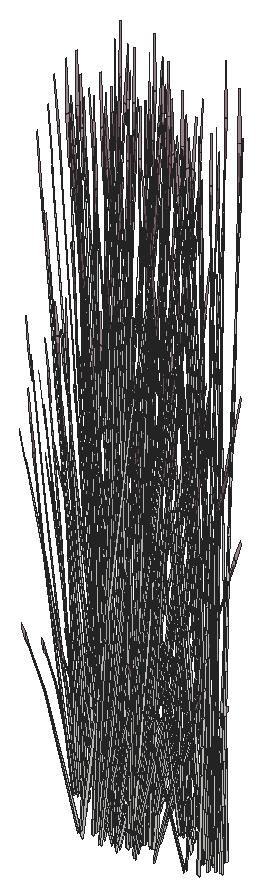
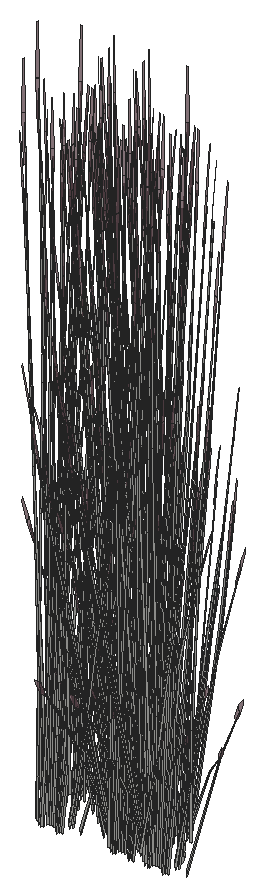
# SketchUp Ruby script. Lengths in inches.
U = 1.inch
M = Sketchup.active_model
def pt(a) = Geom::Point3d.new(a.map { |v| v * U })
def face(e, loops, mat)
  f = e.add_face(loops[0].map { |a| pt(a) })
  loops[1..].each { |l| e.add_face(l.map { |a| pt(a) }).erase! }
  f.material = f.back_material = mat if mat
  f
end
# faces: each face lists its corners as indices into pts; further lists are holes
def faces(e, pts, list, mat = nil) = list.each { |f| face(e, (f[0].is_a?(Array) ? f : [f]).map { |l| l.map { |i| pts[i] } }, mat) }
# xy, xz, yz: faces in a plane at the given z, y or x. An outline is a flat list of corners, or four numbers for a rectangle; further outlines are holes
def ring(l) = l.size == 4 ? [[l[0], l[1]], [l[2], l[1]], [l[2], l[3]], [l[0], l[3]]] : l.each_slice(2).to_a
def flat(e, list, mat, &to3) = list.each { |f| face(e, (f[0].is_a?(Array) ? f : [f]).map { |l| ring(l).map { |u, v| to3.(u, v) } }, mat) }
def xy(e, z, list, mat = nil) = flat(e, list, mat) { |x, y| [x, y, z] }
def xz(e, y, list, mat = nil) = flat(e, list, mat) { |x, z| [x, y, z] }
def yz(e, x, list, mat = nil) = flat(e, list, mat) { |y, z| [x, y, z] }
def lines(e, pts, list) = list.each { |a, b| e.add_line(pt(pts[a]), pt(pts[b])) }
# prism: a flat outline (further loops are holes) pulled along v
def prism(e, loops, v, mat = nil)
  f = face(e, loops, mat); d = Geom::Vector3d.new(v.map { |x| x * U })
  f.pushpull(f.normal.samedirection?(d) ? d.length : -d.length)
end
def box(e, o, s, mat = nil) = prism(e, [[o, [o[0] + s[0], o[1], o[2]], [o[0] + s[0], o[1] + s[1], o[2]], [o[0], o[1] + s[1], o[2]]]], [0, 0, s[2]], mat)
def at(x, y, z, deg = 0) = Geom::Transformation.translation(pt([x, y, z])) * Geom::Transformation.rotation(ORIGIN, Z_AXIS, deg.degrees)
def axes(o, x, y, z) = Geom::Transformation.new([*x, 0, *y, 0, *z, 0, *pt(o).to_a, 1])
def part(name) = M.definitions.add(name)
# library, detail: a bought-in or finely detailed component or shape, given as its bounding box
def library(name, o, s) = part(name).tap { |d| box(d.entities, o, s) }
def detail(e, o, s) = box(e.add_group.entities, o, s)
def put(e, d, t, mat = nil) = e.add_instance(d, t).tap { |i| i.material = mat if mat }
def group(e, t, mat = nil) = e.add_group.tap { |g| g.transformation = t; g.material = mat if mat }.entities
root = M.entities
M.materials.add("LightPink_Translucent").color = [144, 107, 117]
M.materials["LightPink_Translucent"].alpha = 0.75
c1 = part("blade")
p = [[2.15,0.21,22],[0,0.17,0],[0.09,0.45,0],[2.18,0.31,22],[2.29,0.31,22],[0.38,0.45,0],
  [2.48,0.24,33],[2.49,0.24,33],[2.48,0.22,33]]
faces(c1.entities,p,[[0,1,2,3],[4,5,2,3],[6,3,4,7],[8,0,3,6]])
c2 = part("seeds")
p = [[0.3,-0.1,1.38],[-0.01,-0.03,1.59],[-0.01,-0.03,0.03],[0.14,-0.07,-0.07],[0.29,-0.03,3],[0.15,0.01,3.11]]
faces(c2.entities,p,[[0,1,2,3],[1,0,4,5]],"LightPink_Translucent")
c3 = part("blade with seeds")
put(c3.entities,c1,at(0,0,0))
put(c3.entities,c2,axes([2.4,0.25,30.99],[1.5799,-0.05474,1.17369],[-0.12525,1.92788,0.29478],[-0.07173,-0.02425,1.56792]))
put(root,c3,axes([341.09,662.42,620.3],[-0.32829,-0.4014,-0.06131],[0.32849,-0.40164,0],[-0.01146,-0.01402,1.75571]))
put(root,c3,axes([343.38,660.95,620.47],[-0.10196,0.46348,0.17642],[-0.3731,-0.13116,0.35086],[0.06445,-0.00226,1.60407]))
put(root,c3,axes([345.23,662.46,623.05],[-0.29332,-0.1301,0.35414],[0.08555,-0.37955,-0.4572],[0.11809,-0.0348,0.87481]))
put(root,c3,axes([340.27,660.97,620.47],[-0.10196,0.46348,0.17642],[-0.3731,-0.13116,0.35086],[0.06445,-0.00226,1.60407]))
put(root,c3,axes([342.12,662.48,623.05],[-0.29332,-0.1301,0.35414],[0.08555,-0.37955,-0.4572],[0.11809,-0.0348,0.87481]))
put(root,c3,axes([350.53,662.5,620.3],[-0.32829,-0.4014,-0.06131],[0.32849,-0.40164,0],[-0.01146,-0.01402,1.75571]))
put(root,c3,axes([342.16,661.76,622.73],[0.09971,-0.42522,0.48003],[0.32782,0.1454,0.3958],[-0.12892,0.02555,0.9933]))
put(root,c3,axes([343.23,661.32,619.59],[-0.3474,0.18671,1.28929],[-0.11057,-0.53572,0.50096],[0.21332,0.00891,1.46642]))
put(root,c3,axes([349.71,661.05,620.47],[-0.10196,0.46348,0.17642],[-0.3731,-0.13116,0.35086],[0.06445,-0.00226,1.60407]))
put(root,c3,axes([344.16,661.46,620.62],[0.06809,-0.4162,0.1448],[0.33266,0.07225,-0.41347],[0.06054,0.04274,1.26744]))
put(root,c3,axes([339.05,661.78,622.73],[0.09971,-0.42522,0.48003],[0.32782,0.1454,0.3958],[-0.12892,0.02555,0.9933]))
put(root,c3,axes([340.11,661.34,619.59],[-0.3474,0.18671,1.28929],[-0.11057,-0.53572,0.50096],[0.21332,0.00891,1.46642]))
put(root,c3,axes([341.05,661.48,620.62],[0.06809,-0.4162,0.1448],[0.33266,0.07225,-0.41347],[0.06054,0.04274,1.26744]))
put(root,c3,axes([342.14,661.65,622.73],[-0.12963,-0.31798,0.0643],[0.23638,-0.15564,0.50621],[-0.1042,0.03071,0.77189]))
put(root,c3,axes([339.02,661.67,622.73],[-0.12963,-0.31798,0.0643],[0.23638,-0.15564,0.50621],[-0.1042,0.03071,0.77189]))
put(root,c3,axes([343.59,662.45,620.36],[0.44609,0.09826,0.45755],[-0.09078,0.55493,0.17955],[-0.06519,-0.05359,1.58856]))
put(root,c3,axes([348.49,661.86,622.73],[0.09971,-0.42522,0.48003],[0.32782,0.1454,0.3958],[-0.12892,0.02555,0.9933]))
put(root,c3,axes([345.94,662.05,619.49],[-0.01845,-0.0708,1.76342],[0.12793,-0.41416,-0.26939],[0.12905,-0.00596,0.30037]))
put(root,c3,axes([340.47,662.47,620.36],[0.44609,0.09826,0.45755],[-0.09078,0.55493,0.17955],[-0.06519,-0.05359,1.58856]))
put(root,c3,axes([342.83,662.07,619.49],[-0.01845,-0.0708,1.76342],[0.12793,-0.41416,-0.26939],[0.12905,-0.00596,0.30037]))
put(root,c3,axes([342.13,661.98,619.49],[0.00895,0.0735,1.76342],[-0.18044,0.38382,-0.26939],[-0.12817,-0.01935,0.30037]))
put(root,c3,axes([348.46,661.75,622.73],[-0.12963,-0.31798,0.0643],[0.23638,-0.15564,0.50621],[-0.1042,0.03071,0.77189]))
put(root,c3,axes([344.02,661.57,620.72],[-0.21202,-0.39143,0.44739],[0.32115,-0.27564,-0.21531],[0.06861,0.04843,1.43643]))
put(root,c3,axes([339.02,662,619.49],[0.00895,0.0735,1.76342],[-0.18044,0.38382,-0.26939],[-0.12817,-0.01935,0.30037]))
put(root,c3,axes([349.91,662.55,620.36],[0.44609,0.09826,0.45755],[-0.09078,0.55493,0.17955],[-0.06519,-0.05359,1.58856]))
put(root,c3,axes([340.9,661.59,620.72],[-0.21202,-0.39143,0.44739],[0.32115,-0.27564,-0.21531],[0.06861,0.04843,1.43643]))
put(root,c3,axes([342.92,663.36,620.03],[-0.08291,-0.40636,-0.30978],[0.32928,-0.11539,0.30978],[-0.06638,-0.04686,1.38974]))
put(root,c3,axes([348.46,662.08,619.49],[0.00895,0.0735,1.76342],[-0.18044,0.38382,-0.26939],[-0.12817,-0.01935,0.30037]))
put(root,c3,axes([339.81,663.38,620.03],[-0.08291,-0.40636,-0.30978],[0.32928,-0.11539,0.30978],[-0.06638,-0.04686,1.38974]))
put(root,c3,axes([349.25,663.46,620.03],[-0.08291,-0.40636,-0.30978],[0.32928,-0.11539,0.30978],[-0.06638,-0.04686,1.38974]))
put(root,c3,axes([343.35,663.34,620.47],[0.37926,-0.12378,0.17642],[0.09365,0.46065,0.35086],[-0.03382,-0.06712,1.60407]))
put(root,c3,axes([344.125,661.6,620.67],[0.35635,-0.30962,-0.29095],[0.23697,0.43749,-0.50002],[0.08792,0.04443,1.59708]))
put(root,c3,axes([345.54,662.41,622.53],[0.29332,0.1301,-0.35414],[-0.08555,0.37955,0.4572],[0.11809,-0.0348,0.87481]))
put(root,c3,axes([340.23,663.36,620.47],[0.37926,-0.12378,0.17642],[0.09365,0.46065,0.35086],[-0.03382,-0.06712,1.60407]))
put(root,c3,axes([341.01,661.62,620.67],[0.35635,-0.30962,-0.29095],[0.23697,0.43749,-0.50002],[0.08792,0.04443,1.59708]))
put(root,c3,axes([342.43,662.44,622.53],[0.29332,0.1301,-0.35414],[-0.08555,0.37955,0.4572],[0.11809,-0.0348,0.87481]))
put(root,c3,axes([349.67,663.4375,620.47],[0.37926,-0.12378,0.17642],[0.09365,0.46065,0.35086],[-0.03382,-0.06712,1.60407]))
put(root,c3,axes([342.83,663.54,620.02],[-0.33032,-0.23318,-0.49651],[0.19744,-0.41812,0],[-0.07523,-0.05311,1.57504]))
put(root,c3,axes([345.03,660.77,620.02],[0.33032,0.23318,-0.49651],[-0.19744,0.41812,0],[0.07523,0.05311,1.57504]))
put(root,c3,axes([339.72,663.56,620.02],[-0.33032,-0.23318,-0.49651],[0.19744,-0.41812,0],[-0.07523,-0.05311,1.57504]))
put(root,c3,axes([342.1,661.81,622.53],[-0.29332,-0.1301,-0.35414],[0.08555,-0.37955,0.4572],[-0.11809,0.0348,0.87481]))
put(root,c3,axes([341.91,660.8,620.02],[0.33032,0.23318,-0.49651],[-0.19744,0.41812,0],[0.07523,0.05311,1.57504]))
put(root,c3,axes([338.98,661.83,622.53],[-0.29332,-0.1301,-0.35414],[0.08555,-0.37955,0.4572],[-0.11809,0.0348,0.87481]))
put(root,c3,axes([344.4,662.1,620.21],[0.39487,0,0],[0,0.48281,0],[0,0,1.78407]))
put(root,c3,axes([341.28,662.125,620.21],[0.39487,0,0],[0,0.48281,0],[0,0,1.78407]))
put(root,c3,axes([349.15,663.63,620.02],[-0.33032,-0.23318,-0.49651],[0.19744,-0.41812,0],[-0.07523,-0.05311,1.57504]))
put(root,c3,axes([343.73,662.71,620.67],[-0.35635,0.30962,-0.29095],[-0.23697,-0.43749,-0.50002],[-0.08792,-0.04443,1.59708]))
put(root,c3,axes([344.51,660.97,620.47],[-0.37926,0.12378,0.17642],[-0.09365,-0.46065,0.35086],[0.03382,0.06712,1.60407]))
put(root,c3,axes([348.42,661.91,622.53],[-0.29332,-0.1301,-0.35414],[0.08555,-0.37955,0.4572],[-0.11809,0.0348,0.87481]))
put(root,c3,axes([340.61,662.73,620.67],[-0.35635,0.30962,-0.29095],[-0.23697,-0.43749,-0.50002],[-0.08792,-0.04443,1.59708]))
put(root,c3,axes([341.4,660.99,620.47],[-0.37926,0.12378,0.17642],[-0.09365,-0.46065,0.35086],[0.03382,0.06712,1.60407]))
put(root,c3,axes([350.05,662.8125,620.67],[-0.35635,0.30962,-0.29095],[-0.23697,-0.43749,-0.50002],[-0.08792,-0.04443,1.59708]))
put(root,c3,axes([350.83,661.07,620.47],[-0.37926,0.12378,0.17642],[-0.09365,-0.46065,0.35086],[0.03382,0.06712,1.60407]))
put(root,c3,axes([344.74,661.94,621.875],[-0.14639,0.01056,1.71376],[0.09712,-0.45778,0.13857],[0.20862,0.02831,0.73262]))
put(root,c3,axes([341.63,661.97,621.875],[-0.14639,0.01056,1.71376],[0.09712,-0.45778,0.13857],[0.20862,0.02831,0.73262]))
put(root,c3,axes([344.93,660.95,620.03],[0.08291,0.40636,-0.30978],[-0.32928,0.11539,0.30978],[0.06638,0.04686,1.38974]))
put(root,c3,axes([341.82,660.97,620.03],[0.08291,0.40636,-0.30978],[-0.32928,0.11539,0.30978],[0.06638,0.04686,1.38974]))
put(root,c3,axes([345.5,662.57,622.73],[0.12963,0.31798,0.0643],[-0.23638,0.15564,0.50621],[0.1042,-0.03071,0.77189]))
put(root,c3,axes([342.39,662.59,622.73],[0.12963,0.31798,0.0643],[-0.23638,0.15564,0.50621],[0.1042,-0.03071,0.77189]))
put(root,c3,axes([344.27,661.86,620.38],[-0.44609,-0.09826,0.49198],[0.09078,-0.55493,0.19306],[0.06519,0.05359,1.70813]))
put(root,c3,axes([345.48,662.46,622.73],[-0.09971,0.42522,0.48003],[-0.32782,-0.1454,0.3958],[0.12892,-0.02555,0.9933]))
put(root,c3,axes([341.16,661.88,620.38],[-0.44609,-0.09826,0.49198],[0.09078,-0.55493,0.19306],[0.06519,0.05359,1.70813]))
put(root,c3,axes([342.36,662.48,622.73],[-0.09971,0.42522,0.48003],[-0.32782,-0.1454,0.3958],[0.12892,-0.02555,0.9933]))
put(root,c3,axes([343.92,663.23,620.2],[-0.11516,-0.40207,0],[0.32884,-0.1408,0],[0,0,1.54371]))
put(root,c3,axes([340.8,663.25,620.2],[-0.11516,-0.40207,0],[0.32884,-0.1408,0],[0,0,1.54371]))
put(root,c3,axes([343.7,662.85,620.62],[-0.06809,0.4162,0.1448],[-0.33266,-0.07225,-0.41347],[-0.06054,-0.04274,1.26744]))
put(root,c3,axes([342.4,661.77,623.05],[0.29332,0.1301,0.35414],[-0.08555,0.37955,-0.4572],[-0.11809,0.0348,0.87481]))
put(root,c3,axes([340.58,662.87,620.62],[-0.06809,0.4162,0.1448],[-0.33266,-0.07225,-0.41347],[-0.06054,-0.04274,1.26744]))
put(root,c3,axes([339.29,661.79,623.05],[0.29332,0.1301,0.35414],[-0.08555,0.37955,-0.4572],[-0.11809,0.0348,0.87481]))
put(root,c3,axes([350.24,663.33,620.2],[-0.11516,-0.40207,0],[0.32884,-0.1408,0],[0,0,1.54371]))
put(root,c3,axes([344.35,663.17,620.18],[0.37054,-0.15823,-0.19198],[0.1302,0.45581,0.00008],[0.0409,-0.01749,1.73897]))
put(root,c3,axes([341.23,663.19,620.18],[0.37054,-0.15823,-0.19198],[0.1302,0.45581,0.00008],[0.0409,-0.01749,1.73897]))
put(root,c3,axes([350.02,662.95,620.62],[-0.06809,0.4162,0.1448],[-0.33266,-0.07225,-0.41347],[-0.06054,-0.04274,1.26744]))
put(root,c3,axes([344.47,663.36,620.47],[0.10196,-0.46348,0.17642],[0.3731,0.13116,0.35086],[-0.06445,0.00226,1.60407]))
put(root,c3,axes([348.73,661.87,623.05],[0.29332,0.1301,0.35414],[-0.08555,0.37955,-0.4572],[-0.11809,0.0348,0.87481]))
put(root,c3,axes([341.36,663.38,620.47],[0.10196,-0.46348,0.17642],[0.3731,0.13116,0.35086],[-0.06445,0.00226,1.60407]))
put(root,c3,axes([344.39,662.3125,620.21],[0.24637,0.30123,0],[-0.24637,0.30123,0],[0,0,1.69266]))
put(root,c3,axes([341.28,662.33,620.21],[0.24637,0.30123,0],[-0.24637,0.30123,0],[0,0,1.69266]))
put(root,c3,axes([350.8,663.46,620.47],[0.10196,-0.46348,0.17642],[0.3731,0.13116,0.35086],[-0.06445,0.00226,1.60407]))
put(root,c3,axes([342.99,661.75,621.34],[0.10032,-0.06746,1.77064],[0.0346,0.47103,0.13857],[-0.2173,0.0625,0.63284]))
put(root,c3,axes([345.06,662.18,620.47],[-0.2773,-0.3397,0.17642],[0.27945,-0.32949,0.35086],[-0.03063,0.06937,1.60407]))
put(root,c3,axes([339.875,661.77,621.34],[0.10032,-0.06746,1.77064],[0.0346,0.47103,0.13857],[-0.2173,0.0625,0.63284]))
put(root,c3,axes([341.94,662.2,620.47],[-0.2773,-0.3397,0.17642],[0.27945,-0.32949,0.35086],[-0.03063,0.06937,1.60407]))
put(root,c3,axes([344.54,661.67,620.06],[0.36714,0.07646,-0.62353],[-0.07747,0.47163,-0.16365],[0.10956,0.05715,1.37633]))
put(root,c3,axes([346.17,662.49,620.77],[-0.21807,0.07699,1.1486],[0.10265,-0.31819,0.84392],[0.11568,0.02177,0.25299]))
put(root,c3,axes([341.43,661.6875,620.06],[0.36714,0.07646,-0.62353],[-0.07747,0.47163,-0.16365],[0.10956,0.05715,1.37633]))
put(root,c3,axes([343.05,662.51,620.77],[-0.21807,0.07699,1.1486],[0.10265,-0.31819,0.84392],[0.11568,0.02177,0.25299]))
put(root,c3,axes([349.3125,661.85,621.34],[0.10032,-0.06746,1.77064],[0.0346,0.47103,0.13857],[-0.2173,0.0625,0.63284]))
put(root,c3,axes([351.38,662.28,620.47],[-0.2773,-0.3397,0.17642],[0.27945,-0.32949,0.35086],[-0.03063,0.06937,1.60407]))
put(root,c3,axes([343.83,663.41,620.2],[-0.35581,-0.20937,0],[0.17124,-0.43505,0],[0,0,1.62707]))
put(root,c3,axes([344.13,662.85,620.46],[-0.34464,-0.37536,-0.25192],[0.29,-0.42149,0.5513],[-0.0928,0.04391,1.68216]))
put(root,c3,axes([343.22,663.57,620.48],[0.33032,0.23318,0.49651],[-0.19744,0.41812,0],[-0.07523,-0.05311,1.57504]))
put(root,c3,axes([340.72,663.43,620.2],[-0.35581,-0.20937,0],[0.17124,-0.43505,0],[0,0,1.62707]))
put(root,c3,axes([341.01,662.875,620.46],[-0.34464,-0.37536,-0.25192],[0.29,-0.42149,0.5513],[-0.0928,0.04391,1.68216]))
put(root,c3,axes([340.11,663.59,620.48],[0.33032,0.23318,0.49651],[-0.19744,0.41812,0],[-0.07523,-0.05311,1.57504]))
put(root,c3,axes([350.16,663.51,620.2],[-0.35581,-0.20937,0],[0.17124,-0.43505,0],[0,0,1.62707]))
put(root,c3,axes([350.45,662.95,620.46],[-0.34464,-0.37536,-0.25192],[0.29,-0.42149,0.5513],[-0.0928,0.04391,1.68216]))
put(root,c3,axes([349.55,663.67,620.48],[0.33032,0.23318,0.49651],[-0.19744,0.41812,0],[-0.07523,-0.05311,1.57504]))
put(root,c3,axes([344.39,661.96,620.72],[0.17124,-0.42022,0.44739],[0.35581,0.20224,-0.21531],[0,0.09687,1.43643]))
put(root,c3,axes([341.27,661.98,620.72],[0.17124,-0.42022,0.44739],[0.35581,0.20224,-0.21531],[0,0.09687,1.43643]))
put(root,c3,axes([346.0625,663.84,622.71],[-0.03191,-0.04083,1.77383],[0.06981,-0.43764,-0.16761],[0.12571,-0.02796,0.31391]))
put(root,c3,axes([342.95,663.86,622.71],[-0.03191,-0.04083,1.77383],[0.06981,-0.43764,-0.16761],[0.12571,-0.02796,0.31391]))
put(root,c3,axes([341.91,662.0625,622.72],[-0.05763,0.06055,1.74944],[0.0049,0.44239,-0.27667],[-0.13211,0.05753,0.14031]))
put(root,c3,axes([344.32,662.2,620.29],[0,0.53934,-0.05637],[-0.44133,0,0],[0,0.01695,1.79368]))
put(root,c3,axes([342.3,662,622.68],[-0.09562,0.42421,-0.51099],[-0.32782,-0.1454,-0.3958],[-0.13199,0.0389,0.97773]))
put(root,c3,axes([342.28,661.64,623.03],[0.17758,0.42229,-0.1216],[-0.31518,0.20752,-0.67495],[-0.13282,0.05572,1.02557]))
put(root,c3,axes([338.8,662.08,622.72],[-0.05763,0.06055,1.74944],[0.0049,0.44239,-0.27667],[-0.13211,0.05753,0.14031]))
put(root,c3,axes([341.21,662.22,620.29],[0,0.53934,-0.05637],[-0.44133,0,0],[0,0.01695,1.79368]))
put(root,c3,axes([339.18,662.02,622.68],[-0.09562,0.42421,-0.51099],[-0.32782,-0.1454,-0.3958],[-0.13199,0.0389,0.97773]))
put(root,c3,axes([344.35,661.82,620.21],[0.21202,0.39143,-0.44739],[-0.32115,0.27564,0.21531],[0.06861,0.04843,1.43643]))
put(root,c3,axes([339.17,661.66,623.03],[0.17758,0.42229,-0.1216],[-0.31518,0.20752,-0.67495],[-0.13282,0.05572,1.02557]))
put(root,c3,axes([341.24,661.84,620.21],[0.21202,0.39143,-0.44739],[-0.32115,0.27564,0.21531],[0.06861,0.04843,1.43643]))
put(root,c3,axes([345.79,663.47,621.93],[-0.06755,-0.39203,-0.03492],[0.31928,-0.09013,-0.15832],[0.06667,0.02485,0.52218]))
put(root,c3,axes([342.67,663.49,621.93],[-0.06755,-0.39203,-0.03492],[0.31928,-0.09013,-0.15832],[0.06667,0.02485,0.52218]))
put(root,c3,axes([343.03,663.82,620.375],[-0.22066,0.46731,0],[-0.36918,-0.26061,-0.51607],[-0.08408,-0.05936,1.63711]))
put(root,c3,axes([344.96,663.46,623.03],[0.0189,-0.47427,-0.1216],[0.35781,0.01296,-0.67495],[0.13781,0.03295,1.02557]))
put(root,c3,axes([348.23,662.16,622.72],[-0.05763,0.06055,1.74944],[0.0049,0.44239,-0.27667],[-0.13211,0.05753,0.14031]))
put(root,c3,axes([339.92,663.84,620.375],[-0.22066,0.46731,0],[-0.36918,-0.26061,-0.51607],[-0.08408,-0.05936,1.63711]))
put(root,c3,axes([350.64,662.3,620.29],[0,0.53934,-0.05637],[-0.44133,0,0],[0,0.01695,1.79368]))
put(root,c3,axes([348.62,662.1,622.68],[-0.09562,0.42421,-0.51099],[-0.32782,-0.1454,-0.3958],[-0.13199,0.0389,0.97773]))
put(root,c3,axes([341.84,663.48,623.03],[0.0189,-0.47427,-0.1216],[0.35781,0.01296,-0.67495],[0.13781,0.03295,1.02557]))
put(root,c3,axes([348.61,661.74,623.03],[0.17758,0.42229,-0.1216],[-0.31518,0.20752,-0.67495],[-0.13282,0.05572,1.02557]))
put(root,c3,axes([345.29,662.19,620.48],[0,-0.46636,0.49651],[0.39487,0,0],[0,0.10622,1.57504]))
put(root,c3,axes([349.36,663.92,620.375],[-0.22066,0.46731,0],[-0.36918,-0.26061,-0.51607],[-0.08408,-0.05936,1.63711]))
put(root,c3,axes([342.17,662.21,620.48],[0,-0.46636,0.49651],[0.39487,0,0],[0,0.10622,1.57504]))
put(root,c3,axes([344.3,662.54,620.72],[0.38326,-0.02879,0.44739],[0.03466,0.47788,-0.21531],[-0.06861,0.04843,1.43643]))
put(root,c3,axes([344.53,662.06,620.62],[0.32884,-0.136,0.1448],[0.11516,0.38837,-0.41347],[0,0.08547,1.26744]))
put(root,c3,axes([341.18,662.5625,620.72],[0.38326,-0.02879,0.44739],[0.03466,0.47788,-0.21531],[-0.06861,0.04843,1.43643]))
put(root,c3,axes([341.42,662.08,620.62],[0.32884,-0.136,0.1448],[0.11516,0.38837,-0.41347],[0,0.08547,1.26744]))
put(root,c3,axes([344.9,663.27,623.05],[-0.20082,-0.29199,0.35414],[0.2293,-0.2764,-0.4572],[0.1165,0.04206,0.87481]))
put(root,c3,axes([350.62,662.64,620.72],[0.38326,-0.02879,0.44739],[0.03466,0.47788,-0.21531],[-0.06861,0.04843,1.43643]))
put(root,c3,axes([341.79,663.3,623.05],[-0.20082,-0.29199,0.35414],[0.2293,-0.2764,-0.4572],[0.1165,0.04206,0.87481]))
put(root,c3,axes([343.95,662.77,620.21],[-0.38326,0.02879,-0.44739],[-0.03466,-0.47788,0.21531],[-0.06861,0.04843,1.43643]))
put(root,c3,axes([340.84,662.79,620.21],[-0.38326,0.02879,-0.44739],[-0.03466,-0.47788,0.21531],[-0.06861,0.04843,1.43643]))
put(root,c3,axes([345.76,663,620.59],[-0.085,-0.1147,1.43002],[0.1106,-0.37943,-0.30754],[0.17198,0.0514,0.61141]))
put(root,c3,axes([350.28,662.875,620.21],[-0.38326,0.02879,-0.44739],[-0.03466,-0.47788,0.21531],[-0.06861,0.04843,1.43643]))
put(root,c3,axes([342.64,663.02,620.59],[-0.085,-0.1147,1.43002],[0.1106,-0.37943,-0.30754],[0.17198,0.0514,0.61141]))
put(root,c3,axes([344.24,663.42,620.2],[0.35581,0.20937,0],[-0.17124,0.43505,0],[0,0,1.74954]))
put(root,c3,axes([341.125,663.44,620.2],[0.35581,0.20937,0],[-0.17124,0.43505,0],[0,0,1.74954]))
put(root,c3,axes([345.27,663.18,622.72],[0.07571,-0.00789,1.74944],[0.20767,-0.36231,-0.27667],[0.13467,0.04783,0.14031]))
put(root,c3,axes([344.38,663.88,620.19],[-0.21791,-0.46895,-0.05142],[0.36918,-0.26061,0.51607],[-0.09097,0.04465,1.6363]))
put(root,c3,axes([342.16,663.2,622.72],[0.07571,-0.00789,1.74944],[0.20767,-0.36231,-0.27667],[0.13467,0.04783,0.14031]))
put(root,c3,axes([341.26,663.9,620.19],[-0.21791,-0.46895,-0.05142],[0.36918,-0.26061,0.51607],[-0.09097,0.04465,1.6363]))
put(root,c3,axes([344.3,662.75,620.62],[0.26075,0.2802,0.1448],[-0.2175,0.31612,-0.41347],[-0.06054,0.04274,1.26744]))
put(root,c3,axes([341.1875,662.77,620.62],[0.26075,0.2802,0.1448],[-0.2175,0.31612,-0.41347],[-0.06054,0.04274,1.26744]))
put(root,c3,axes([342.24,662.82,622.73],[-0.08753,-0.42921,0.48003],[0.34336,-0.07449,0.3958],[-0.1012,0.10094,0.9933]))
put(root,c3,axes([342.18,662.74,622.73],[-0.2423,-0.19613,0.0643],[0.14107,-0.2793,0.50621],[-0.07768,0.0903,0.77189]))
put(root,c3,axes([339.13,662.84,622.73],[-0.08753,-0.42921,0.48003],[0.34336,-0.07449,0.3958],[-0.1012,0.10094,0.9933]))
put(root,c3,axes([342.29,662.22,621.875],[0.12246,-0.09864,1.71376],[0.1031,0.45582,0.13857],[-0.19225,0.10302,0.73262]))
put(root,c3,axes([339.0625,662.76,622.73],[-0.2423,-0.19613,0.0643],[0.14107,-0.2793,0.50621],[-0.07768,0.0903,0.77189]))
put(root,c3,axes([350.7,663.98,620.19],[-0.21791,-0.46895,-0.05142],[0.36918,-0.26061,0.51607],[-0.09097,0.04465,1.6363]))
put(root,c3,axes([339.17,662.24,621.875],[0.12246,-0.09864,1.71376],[0.1031,0.45582,0.13857],[-0.19225,0.10302,0.73262]))
put(root,c3,axes([350.625,662.85,620.62],[0.26075,0.2802,0.1448],[-0.2175,0.31612,-0.41347],[-0.06054,0.04274,1.26744]))
put(root,c3,axes([348.57,662.92,622.73],[-0.08753,-0.42921,0.48003],[0.34336,-0.07449,0.3958],[-0.1012,0.10094,0.9933]))
put(root,c3,axes([348.5,662.84,622.73],[-0.2423,-0.19613,0.0643],[0.14107,-0.2793,0.50621],[-0.07768,0.0903,0.77189]))
put(root,c3,axes([348.61,662.32,621.875],[0.12246,-0.09864,1.71376],[0.1031,0.45582,0.13857],[-0.19225,0.10302,0.73262]))
put(root,c3,axes([344.98,663.23,622.98],[0.35281,0.01123,-0.71045],[-0.0237,0.47284,0.08574],[0.14947,0.0499,1.00501]))
put(root,c3,axes([341.86,663.25,622.98],[0.35281,0.01123,-0.71045],[-0.0237,0.47284,0.08574],[0.14947,0.0499,1.00501]))
put(root,c3,axes([344.58,663.61,620.48],[0.33032,-0.23318,0.49651],[0.19744,0.41812,0],[-0.07523,0.05311,1.57504]))
put(root,c3,axes([341.46,663.63,620.48],[0.33032,-0.23318,0.49651],[0.19744,0.41812,0],[-0.07523,0.05311,1.57504]))
put(root,c3,axes([344.11,663.24,620.29],[0.15345,0.53576,-0.06012],[-0.43845,0.18773,0],[0.00536,0.01871,1.72173]))
put(root,c3,axes([341,663.26,620.29],[0.15345,0.53576,-0.06012],[-0.43845,0.18773,0],[0.00536,0.01871,1.72173]))
put(root,c3,axes([344.28,663.82,620.03],[-0.32928,-0.11539,-0.30978],[0.08291,-0.40636,0.30978],[-0.06638,0.04686,1.38974]))
put(root,c3,axes([350.9,663.71,620.48],[0.33032,-0.23318,0.49651],[0.19744,0.41812,0],[-0.07523,0.05311,1.57504]))
put(root,c3,axes([341.17,663.84,620.03],[-0.32928,-0.11539,-0.30978],[0.08291,-0.40636,0.30978],[-0.06638,0.04686,1.38974]))
put(root,c3,axes([341.9,663,620.59],[0.12266,0.03828,1.43002],[0.07906,0.39104,-0.30754],[-0.16661,0.0732,0.61141]))
put(root,c3,axes([338.79,663.02,620.59],[0.12266,0.03828,1.43002],[0.07906,0.39104,-0.30754],[-0.16661,0.0732,0.61141]))
put(root,c3,axes([350.43,663.34,620.29],[0.15345,0.53576,-0.06012],[-0.43845,0.18773,0],[0.00536,0.01871,1.72173]))
put(root,c3,axes([342.45,662.68,623.05],[0.30722,-0.06665,0.35414],[0.08112,0.381,-0.4572],[-0.08804,0.10234,0.87481]))
put(root,c3,axes([350.6,663.92,620.03],[-0.32928,-0.11539,-0.30978],[0.08291,-0.40636,0.30978],[-0.06638,0.04686,1.38974]))
put(root,c3,axes([345.55,662.27,620.375],[0.44133,0,0],[0,0.52122,-0.51607],[0,0.11871,1.63711]))
put(root,c3,axes([339.34,662.7,623.05],[0.30722,-0.06665,0.35414],[0.08112,0.381,-0.4572],[-0.08804,0.10234,0.87481]))
put(root,c3,axes([342.4375,662.29,620.375],[0.44133,0,0],[0,0.52122,-0.51607],[0,0.11871,1.63711]))
put(root,c3,axes([348.23,663.1,620.59],[0.12266,0.03828,1.43002],[0.07906,0.39104,-0.30754],[-0.16661,0.0732,0.61141]))
put(root,c3,axes([341.27,662.51,622.71],[0.04504,0.01251,1.77383],[0.13934,0.41205,-0.16761],[-0.0922,0.10815,0.31391]))
put(root,c3,axes([345.375,662.54,620.2],[-0.44111,-0.00373,-0.04976],[0,-0.52122,0.49943],[-0.01386,0.11865,1.58352]))
put(root,c3,axes([338.16,662.53,622.71],[0.04504,0.01251,1.77383],[0.13934,0.41205,-0.16761],[-0.0922,0.10815,0.31391]))
put(root,c3,axes([344.42,662.09,620.67],[0.39748,0.22252,-0.29095],[-0.19139,0.46966,-0.50002],[0.01249,0.11531,1.59708]))
put(root,c3,axes([342.26,662.5625,620.2],[-0.44111,-0.00373,-0.04976],[0,-0.52122,0.49943],[-0.01386,0.11865,1.58352]))
put(root,c3,axes([348.78,662.78,623.05],[0.30722,-0.06665,0.35414],[0.08112,0.381,-0.4572],[-0.08804,0.10234,0.87481]))
put(root,c3,axes([341.31,662.11,620.67],[0.39748,0.22252,-0.29095],[-0.19139,0.46966,-0.50002],[0.01249,0.11531,1.59708]))
put(root,c3,axes([341.65,663.82,620.77],[0.14709,-0.21136,1.1486],[0.05804,0.3346,0.84392],[-0.1063,0.05991,0.25299]))
put(root,c3,axes([345.1875,663.43,622.53],[0.20082,0.29199,-0.35414],[-0.2293,0.2764,0.4572],[0.1165,0.04206,0.87481]))
put(root,c3,axes([347.59,662.61,622.71],[0.04504,0.01251,1.77383],[0.13934,0.41205,-0.16761],[-0.0922,0.10815,0.31391]))
put(root,c3,axes([345.29,662.62,620.03],[-0.24637,0.29097,-0.30978],[-0.24637,-0.29097,0.30978],[0,0.09372,1.38974]))
put(root,c3,axes([351.7,662.64,620.2],[-0.44111,-0.00373,-0.04976],[0,-0.52122,0.49943],[-0.01386,0.11865,1.58352]))
put(root,c3,axes([338.53,663.84,620.77],[0.14709,-0.21136,1.1486],[0.05804,0.3346,0.84392],[-0.1063,0.05991,0.25299]))
put(root,c3,axes([342.07,663.45,622.53],[0.20082,0.29199,-0.35414],[-0.2293,0.2764,0.4572],[0.1165,0.04206,0.87481]))
put(root,c3,axes([342.17,662.64,620.03],[-0.24637,0.29097,-0.30978],[-0.24637,-0.29097,0.30978],[0,0.09372,1.38974]))
put(root,c3,axes([344.22,662.64,620.67],[0.04113,0.53214,-0.29095],[-0.42835,0.03218,-0.50002],[-0.07543,0.07088,1.59708]))
put(root,c3,axes([345.09,663.54,622.73],[-0.01777,0.35463,0.0643],[-0.26836,-0.00972,0.50621],[0.1028,0.03711,0.77189]))
put(root,c3,axes([341.11,662.67,620.67],[0.04113,0.53214,-0.29095],[-0.42835,0.03218,-0.50002],[-0.07543,0.07088,1.59708]))
put(root,c3,axes([341.97,663.56,622.73],[-0.01777,0.35463,0.0643],[-0.26836,-0.00972,0.50621],[0.1028,0.03711,0.77189]))
put(root,c3,axes([344.38,662.4375,620.21],[-0.17124,0.42022,-0.44739],[-0.35581,-0.20224,0.21531],[0,0.09687,1.43643]))
put(root,c3,axes([347.97,663.92,620.77],[0.14709,-0.21136,1.1486],[0.05804,0.3346,0.84392],[-0.1063,0.05991,0.25299]))
